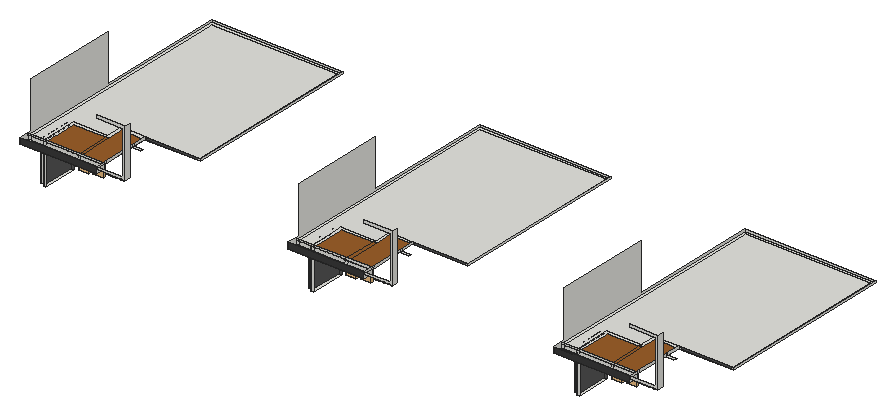
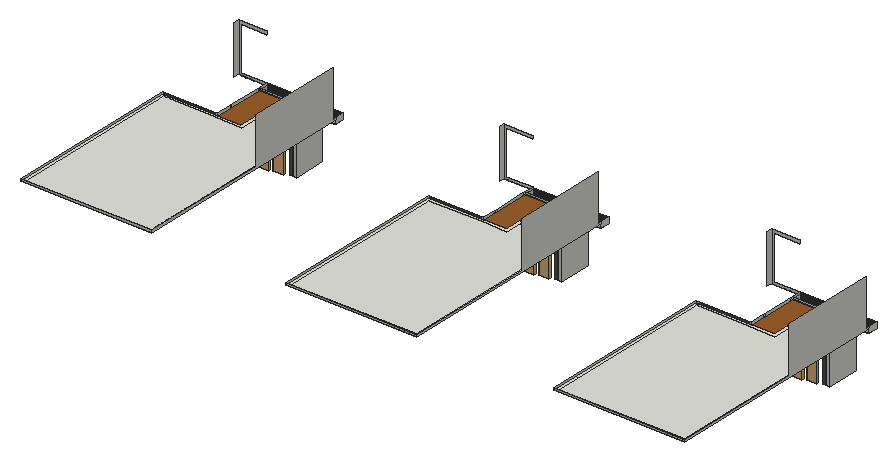
# SketchUp Ruby script. Lengths in inches.
U = 1.inch
M = Sketchup.active_model
def pt(a) = Geom::Point3d.new(a.map { |v| v * U })
def face(e, loops, mat)
  f = e.add_face(loops[0].map { |a| pt(a) })
  loops[1..].each { |l| e.add_face(l.map { |a| pt(a) }).erase! }
  f.material = f.back_material = mat if mat
  f
end
# faces: each face lists its corners as indices into pts; further lists are holes
def faces(e, pts, list, mat = nil) = list.each { |f| face(e, (f[0].is_a?(Array) ? f : [f]).map { |l| l.map { |i| pts[i] } }, mat) }
# xy, xz, yz: faces in a plane at the given z, y or x. An outline is a flat list of corners, or four numbers for a rectangle; further outlines are holes
def ring(l) = l.size == 4 ? [[l[0], l[1]], [l[2], l[1]], [l[2], l[3]], [l[0], l[3]]] : l.each_slice(2).to_a
def flat(e, list, mat, &to3) = list.each { |f| face(e, (f[0].is_a?(Array) ? f : [f]).map { |l| ring(l).map { |u, v| to3.(u, v) } }, mat) }
def xy(e, z, list, mat = nil) = flat(e, list, mat) { |x, y| [x, y, z] }
def xz(e, y, list, mat = nil) = flat(e, list, mat) { |x, z| [x, y, z] }
def yz(e, x, list, mat = nil) = flat(e, list, mat) { |y, z| [x, y, z] }
def lines(e, pts, list) = list.each { |a, b| e.add_line(pt(pts[a]), pt(pts[b])) }
# prism: a flat outline (further loops are holes) pulled along v
def prism(e, loops, v, mat = nil)
  f = face(e, loops, mat); d = Geom::Vector3d.new(v.map { |x| x * U })
  f.pushpull(f.normal.samedirection?(d) ? d.length : -d.length)
end
def box(e, o, s, mat = nil) = prism(e, [[o, [o[0] + s[0], o[1], o[2]], [o[0] + s[0], o[1] + s[1], o[2]], [o[0], o[1] + s[1], o[2]]]], [0, 0, s[2]], mat)
def at(x, y, z, deg = 0) = Geom::Transformation.translation(pt([x, y, z])) * Geom::Transformation.rotation(ORIGIN, Z_AXIS, deg.degrees)
def axes(o, x, y, z) = Geom::Transformation.new([*x, 0, *y, 0, *z, 0, *pt(o).to_a, 1])
def part(name) = M.definitions.add(name)
# library, detail: a bought-in or finely detailed component or shape, given as its bounding box
def library(name, o, s) = part(name).tap { |d| box(d.entities, o, s) }
def detail(e, o, s) = box(e.add_group.entities, o, s)
def put(e, d, t, mat = nil) = e.add_instance(d, t).tap { |i| i.material = mat if mat }
def group(e, t, mat = nil) = e.add_group.tap { |g| g.transformation = t; g.material = mat if mat }.entities
root = M.entities
M.materials.add("[Color M04]").color = [142, 142, 142]
M.materials.add("[Color M06]").color = [86, 86, 86]
M.materials.add("[Color M07]").color = [58, 58, 58]
M.materials.add("[Wood Floor Dark]").color = [153, 94, 42]
c1 = library("Group\#1",[0,0,0],[29.75,5.78,110.95])
xy(root,275.45,[[919.21,302.38,927.52,403.18],[1705.58,302.38,1713.9,403.18],[2485.96,302.38,2494.27,403.18],[907.08,309.31,919.21,403.18],[1693.46,309.31,1705.58,403.18],
  [2473.83,309.31,2485.96,403.18]])
xy(root,357.625,[[938.52,405,1006.52,413.31],[1724.89,405,1792.89,413.31],[2505.27,405,2573.27,413.31]])
xy(root,358.5,[[1084.66,452.97,1043.3,454.25,1043.56,462.56,1084.91,461.29],[1871.03,452.97,1829.68,454.25,1829.93,462.56,1871.29,461.29],[2651.41,452.97,2610.05,454.25,2610.31,462.56,2651.66,461.29]])
xy(root,380.87,[[919.21,302.38,927.52,302.82],[1705.58,302.38,1713.9,302.82],[2485.96,302.38,2494.27,302.82]])
xy(root,382.28,[[902.25,297.375,905.86,300.5625],[907.28,297.375,910.89,300.5625],[911.84,297.375,915.46,300.5625],[916.32,297.375,919.9375,300.5625],[920.81,297.375,924.42,300.5625],
  [1688.62,297.375,1692.23,300.5625],[1693.66,297.375,1697.27,300.5625],[1698.22,297.375,1701.83,300.5625],[1702.7,297.375,1706.3125,300.5625],[1707.18,297.375,1710.79,300.5625],
  [2469,297.375,2472.61,300.5625],[2474.03,297.375,2477.64,300.5625],[2478.59,297.375,2482.21,300.5625],[2483.07,297.375,2486.6875,300.5625],[2487.56,297.375,2491.17,300.5625]])
xy(root,382.6875,[[874.71,297.375,878.33,301],[879.21,297.375,882.83,301],[883.71,297.375,887.33,301],[888.21,297.375,891.83,301],[892.71,297.375,896.33,301],
  [897.21,297.375,900.83,301],[1661.09,297.375,1664.7,301],[1665.59,297.375,1669.2,301],[1670.09,297.375,1673.7,301],[1674.59,297.375,1678.2,301],
  [1679.09,297.375,1682.7,301],[1683.59,297.375,1687.2,301],[2441.46,297.375,2445.08,301],[2445.96,297.375,2449.58,301],[2450.46,297.375,2454.08,301],
  [2454.96,297.375,2458.58,301],[2459.46,297.375,2463.08,301],[2463.96,297.375,2467.58,301],[900.83,300.5625,919.21,301],[919.21,300.5625,927.52,301],
  [1687.2,300.5625,1705.58,301],[1705.58,300.5625,1713.9,301],[2467.58,300.5625,2485.96,301],[2485.96,300.5625,2494.27,301]])
xy(root,382.6875,[[874.71,273.0625,874.71,297.375,878.33,297.375,878.33,301,879.21,301,879.21,297.375,882.83,297.375,882.83,301,883.71,301,883.71,297.375,887.33,297.375,887.33,301,888.21,301,888.21,297.375,891.83,297.375,891.83,301,892.71,301,892.71,297.375,896.33,297.375,896.33,301,897.21,301,897.21,297.375,900.83,297.375,900.83,300.5625,927.52,300.5625,927.52,301,1098.03,301,1098.03,273.0625],[1661.09,273.0625,1661.09,297.375,1664.7,297.375,1664.7,301,1665.59,301,1665.59,297.375,1669.2,297.375,1669.2,301,1670.09,301,1670.09,297.375,1673.7,297.375,1673.7,301,1674.59,301,1674.59,297.375,1678.2,297.375,1678.2,301,1679.09,301,1679.09,297.375,1682.7,297.375,1682.7,301,1683.59,301,1683.59,297.375,1687.2,297.375,1687.2,300.5625,1713.9,300.5625,1713.9,301,1884.4,301,1884.4,273.0625],[2441.46,273.0625,2441.46,297.375,2445.08,297.375,2445.08,301,2445.96,301,2445.96,297.375,2449.58,297.375,2449.58,301,2450.46,301,2450.46,297.375,2454.08,297.375,2454.08,301,2454.96,301,2454.96,297.375,2458.58,297.375,2458.58,301,2459.46,301,2459.46,297.375,2463.08,297.375,2463.08,301,2463.96,301,2463.96,297.375,2467.58,297.375,2467.58,300.5625,2494.27,300.5625,2494.27,301,2664.78,301,2664.78,273.0625]],"[Color M07]")
xy(root,391.8,[[907.08,309.31,919.21,403.18],[1693.46,309.31,1705.58,403.18],[2473.83,309.31,2485.96,403.18]])
xy(root,391.8,[[919.21,302.82,927.52,403.18],[1705.58,302.82,1713.9,403.18],[2485.96,302.82,2494.27,403.18]],"[Wood Floor Dark]")
xy(root,393.625,[[1129.29,271.6875,1141.72,273.0625],[1143.3,271.6875,1155.73,273.0625],[1157.32,271.6875,1169.74,273.0625],[1171.33,271.6875,1181.97,273.0625],[1915.67,271.6875,1928.09,273.0625],
  [1929.68,271.6875,1942.11,273.0625],[1943.69,271.6875,1956.12,273.0625],[1957.7,271.6875,1968.34,273.0625],[2696.04,271.6875,2708.47,273.0625],[2710.05,271.6875,2722.48,273.0625],
  [2724.07,271.6875,2736.49,273.0625],[2738.08,271.6875,2748.72,273.0625],[874.71,301,883.03,301,883.03,967.62,1252.27,967.62,1252.27,460.88,1098.16,460.88,1020.71,463.26,1020.71,405,1029.02,405,1029.02,454.6875,1098.03,452.5625,1260.59,452.5625,1260.59,975.9375,874.71,975.9375],[883.03,301,919.21,309.31],[919.21,301,927.52,301,927.52,405,1020.71,405,1020.71,413.31,919.21,413.31],
  [1661.09,301,1669.4,301,1669.4,967.62,2038.65,967.62,2038.65,460.88,1884.53,460.88,1807.08,463.26,1807.08,405,1815.4,405,1815.4,454.6875,1884.4,452.5625,2046.96,452.5625,2046.96,975.9375,1661.09,975.9375],[1669.4,301,1705.58,309.31],[1705.58,301,1713.9,301,1713.9,405,1807.08,405,1807.08,413.31,1705.58,413.31],[2441.46,301,2449.78,301,2449.78,967.62,2819.02,967.62,2819.02,460.88,2664.91,460.88,2587.46,463.26,2587.46,405,2595.77,405,2595.77,454.6875,2664.78,452.5625,2827.34,452.5625,2827.34,975.9375,2441.46,975.9375],[2449.78,301,2485.96,309.31],
  [2485.96,301,2494.27,301,2494.27,405,2587.46,405,2587.46,413.31,2485.96,413.31],[883.03,309.31,883.03,967.62,1252.27,967.62,1252.27,460.88,1098.16,460.88,1020.71,463.26,1020.71,413.31,919.21,413.31,919.21,309.31],[1669.4,309.31,1669.4,967.62,2038.65,967.62,2038.65,460.88,1884.53,460.88,1807.08,463.26,1807.08,413.31,1705.58,413.31,1705.58,309.31],[2449.78,309.31,2449.78,967.62,2819.02,967.62,2819.02,460.88,2664.91,460.88,2587.46,463.26,2587.46,413.31,2485.96,413.31,2485.96,309.31]])
xy(root,393.625,[[927.52,301,1020.71,405],[1020.71,301,1029.02,405],[1029.02,301,1029.02,454.6875,1098.03,452.5625,1098.03,301],[1713.9,301,1807.08,405],[1807.08,301,1815.4,405],
  [1815.4,301,1815.4,454.6875,1884.4,452.5625,1884.4,301],[2494.27,301,2587.46,405],[2587.46,301,2595.77,405],[2595.77,301,2595.77,454.6875,2664.78,452.5625,2664.78,301]],"[Wood Floor Dark]")
xz(root,273.0625,[[1098.03,393.625,1181.97,393.625,1181.97,536.4375,1098.03,536.4375,1098.03,528.11,1175.84,528.11,1175.84,400.68,1098.03,400.68],[1884.4,393.625,1968.34,393.625,1968.34,536.4375,1884.4,536.4375,1884.4,528.11,1962.22,528.11,1962.22,400.68,1884.4,400.68],[2664.78,393.625,2748.72,393.625,2748.72,536.4375,2664.78,536.4375,2664.78,528.11,2742.59,528.11,2742.59,400.68,2664.78,400.68]])
xz(root,273.0625,[[874.71,382.6875,1098.03,382.6875,1098.03,399.625,933.87,399.625,933.87,399.3125,874.71,399.3125],[1661.09,382.6875,1884.4,382.6875,1884.4,399.625,1720.25,399.625,1720.25,399.3125,1661.09,399.3125],[2441.46,382.6875,2664.78,382.6875,2664.78,399.625,2500.62,399.625,2500.62,399.3125,2441.46,399.3125]],"[Color M07]")
xz(root,301,[[874.71,382.6875,883.03,393.625],[883.03,382.6875,919.21,393.625],[919.21,382.6875,927.52,393.625],[927.52,382.6875,1020.71,393.625],[1020.71,382.6875,1029.02,393.625],
  [1029.02,382.6875,1098.03,393.625],[1661.09,382.6875,1669.4,393.625],[1669.4,382.6875,1705.58,393.625],[1705.58,382.6875,1713.9,393.625],[1713.9,382.6875,1807.08,393.625],
  [1807.08,382.6875,1815.4,393.625],[1815.4,382.6875,1884.4,393.625],[2441.46,382.6875,2449.78,393.625],[2449.78,382.6875,2485.96,393.625],[2485.96,382.6875,2494.27,393.625],
  [2494.27,382.6875,2587.46,393.625],[2587.46,382.6875,2595.77,393.625],[2595.77,382.6875,2664.78,393.625],[874.71,393.625,874.71,399.3125,933.87,399.3125,933.87,399.625,1098.03,399.625,1098.03,393.625],[1661.09,393.625,1661.09,399.3125,1720.25,399.3125,1720.25,399.625,1884.4,399.625,1884.4,393.625],
  [2441.46,393.625,2441.46,399.3125,2500.62,399.3125,2500.62,399.625,2664.78,399.625,2664.78,393.625]])
xz(root,302.38,[[919.21,275.45,927.52,380.87],[1705.58,275.45,1713.9,380.87],[2485.96,275.45,2494.27,380.87]])
xz(root,302.82,[[919.21,380.87,927.52,391.8],[1705.58,380.87,1713.9,391.8],[2485.96,380.87,2494.27,391.8]])
xz(root,309.31,[[907.08,275.45,919.21,391.8],[1693.46,275.45,1705.58,391.8],[2473.83,275.45,2485.96,391.8]])
xz(root,403.18,[[907.08,275.45,919.21,391.8],[1693.46,275.45,1705.58,391.8],[2473.83,275.45,2485.96,391.8]])
xz(root,403.18,[[919.21,275.45,927.52,391.8],[1705.58,275.45,1713.9,391.8],[2485.96,275.45,2494.27,391.8]],"[Color M06]")
xz(root,452.5625,[[1098.03,393.625,1103.7,399.625],[1253.34,393.625,1260.59,399.625],[1884.4,393.625,1890.08,399.625],[2039.72,393.625,2046.96,399.625],[2664.78,393.625,2670.45,399.625],
  [2820.09,393.625,2827.34,399.625]])
xz(root,452.5625,[[1103.7,393.625,1253.34,399.625],[1890.08,393.625,2039.72,399.625],[2670.45,393.625,2820.09,399.625]],"[Color M06]")
xz(root,975.9375,[[874.71,393.625,1260.59,399.625],[1661.09,393.625,2046.96,399.625],[2441.46,393.625,2827.34,399.625]])
yz(root,874.71,[[273.0625,382.6875,301,399.3125],[301,393.625,301,399.3125,311.64,399.3125,311.64,536.4375,593.65,536.4375,593.65,399.625,975.9375,399.625,975.9375,393.625]])
yz(root,907.08,[[309.31,275.45,403.18,391.8]])
yz(root,919.21,[[302.38,275.45,309.31,275.45,309.31,391.8,302.82,391.8,302.82,380.87,302.38,380.87]])
yz(root,919.21,[[309.31,275.45,403.18,391.8]],"[Color M06]")
yz(root,1098.03,[[273.0625,382.6875,301,393.625],[273.0625,393.625,301,399.625],[301,393.625,308.24,399.625],[308.24,393.625,405,399.625],[405,393.625,411.0625,399.625],
  [411.0625,393.625,452.5625,399.625]])
yz(root,1181.97,[[273.0625,393.625,289.5,536.4375]])
yz(root,1260.59,[[452.5625,393.625,975.9375,399.625]])
yz(root,1661.09,[[273.0625,382.6875,301,399.3125],[301,393.625,301,399.3125,311.64,399.3125,311.64,536.4375,593.65,536.4375,593.65,399.625,975.9375,399.625,975.9375,393.625]])
yz(root,1693.46,[[309.31,275.45,403.18,391.8]])
yz(root,1705.58,[[302.38,275.45,309.31,275.45,309.31,391.8,302.82,391.8,302.82,380.87,302.38,380.87]])
yz(root,1705.58,[[309.31,275.45,403.18,391.8]],"[Color M06]")
yz(root,1884.4,[[273.0625,382.6875,301,393.625],[273.0625,393.625,301,399.625],[301,393.625,308.24,399.625],[308.24,393.625,405,399.625],[405,393.625,411.0625,399.625],
  [411.0625,393.625,452.5625,399.625]])
yz(root,1968.34,[[273.0625,393.625,289.5,536.4375]])
yz(root,2046.96,[[452.5625,393.625,975.9375,399.625]])
yz(root,2441.46,[[273.0625,382.6875,301,399.3125],[301,393.625,301,399.3125,311.64,399.3125,311.64,536.4375,593.65,536.4375,593.65,399.625,975.9375,399.625,975.9375,393.625]])
yz(root,2473.83,[[309.31,275.45,403.18,391.8]])
yz(root,2485.96,[[302.38,275.45,309.31,275.45,309.31,391.8,302.82,391.8,302.82,380.87,302.38,380.87]])
yz(root,2485.96,[[309.31,275.45,403.18,391.8]],"[Color M06]")
yz(root,2664.78,[[273.0625,382.6875,301,393.625],[273.0625,393.625,301,399.625],[301,393.625,308.24,399.625],[308.24,393.625,405,399.625],[405,393.625,411.0625,399.625],
  [411.0625,393.625,452.5625,399.625]])
yz(root,2748.72,[[273.0625,393.625,289.5,536.4375]])
yz(root,2827.34,[[452.5625,393.625,975.9375,399.625]])
put(root,c1,axes([1763.14,413.31,276.5625],[1,0,0],[0,1,0],[0,0,0.73062]),"[Color M04]")
put(root,c1,axes([976.77,413.31,276.5625],[1,0,0],[0,1,0],[0,0,0.73062]),"[Color M04]")
put(root,c1,axes([2543.52,413.31,276.5625],[1,0,0],[0,1,0],[0,0,0.73062]),"[Color M04]")
put(root,c1,axes([1723.17,408.72,276.5625],[1,0,0],[0,1,0],[0,0,0.73062]),"[Color M04]")
put(root,c1,axes([936.79,408.72,276.5625],[1,0,0],[0,1,0],[0,0,0.73062]),"[Color M04]")
put(root,c1,axes([2503.54,408.72,276.5625],[1,0,0],[0,1,0],[0,0,0.73062]),"[Color M04]")
